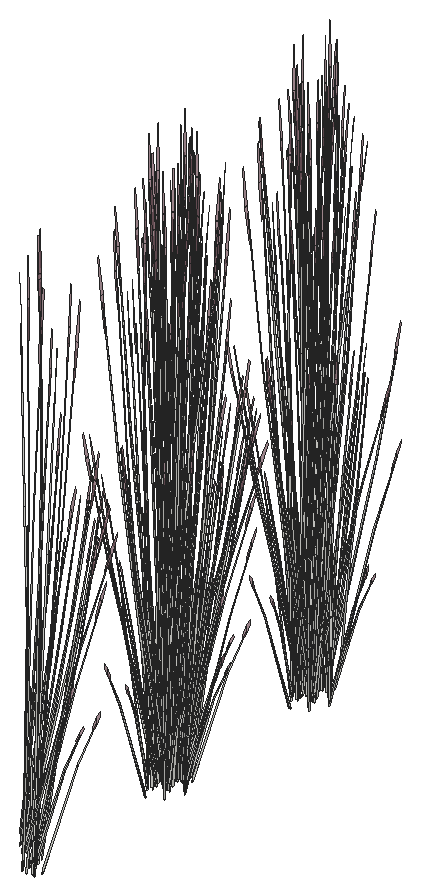
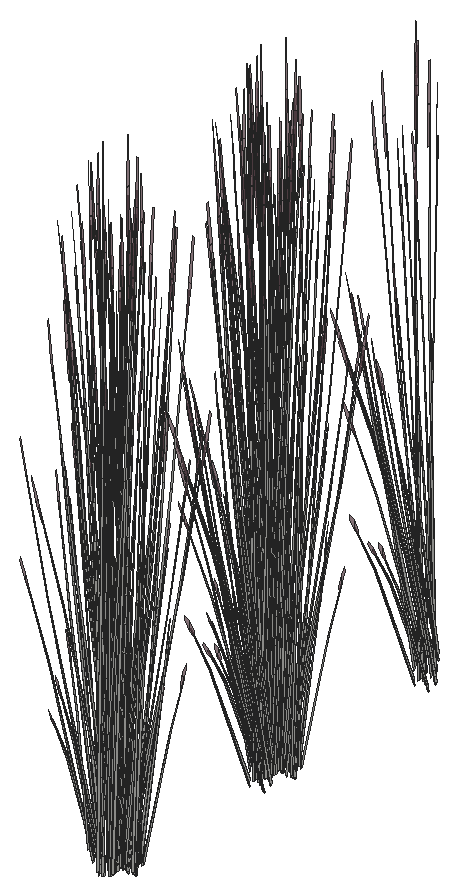
# SketchUp Ruby script. Lengths in inches.
U = 1.inch
M = Sketchup.active_model
def pt(a) = Geom::Point3d.new(a.map { |v| v * U })
def face(e, loops, mat)
  f = e.add_face(loops[0].map { |a| pt(a) })
  loops[1..].each { |l| e.add_face(l.map { |a| pt(a) }).erase! }
  f.material = f.back_material = mat if mat
  f
end
# faces: each face lists its corners as indices into pts; further lists are holes
def faces(e, pts, list, mat = nil) = list.each { |f| face(e, (f[0].is_a?(Array) ? f : [f]).map { |l| l.map { |i| pts[i] } }, mat) }
# xy, xz, yz: faces in a plane at the given z, y or x. An outline is a flat list of corners, or four numbers for a rectangle; further outlines are holes
def ring(l) = l.size == 4 ? [[l[0], l[1]], [l[2], l[1]], [l[2], l[3]], [l[0], l[3]]] : l.each_slice(2).to_a
def flat(e, list, mat, &to3) = list.each { |f| face(e, (f[0].is_a?(Array) ? f : [f]).map { |l| ring(l).map { |u, v| to3.(u, v) } }, mat) }
def xy(e, z, list, mat = nil) = flat(e, list, mat) { |x, y| [x, y, z] }
def xz(e, y, list, mat = nil) = flat(e, list, mat) { |x, z| [x, y, z] }
def yz(e, x, list, mat = nil) = flat(e, list, mat) { |y, z| [x, y, z] }
def lines(e, pts, list) = list.each { |a, b| e.add_line(pt(pts[a]), pt(pts[b])) }
# prism: a flat outline (further loops are holes) pulled along v
def prism(e, loops, v, mat = nil)
  f = face(e, loops, mat); d = Geom::Vector3d.new(v.map { |x| x * U })
  f.pushpull(f.normal.samedirection?(d) ? d.length : -d.length)
end
def box(e, o, s, mat = nil) = prism(e, [[o, [o[0] + s[0], o[1], o[2]], [o[0] + s[0], o[1] + s[1], o[2]], [o[0], o[1] + s[1], o[2]]]], [0, 0, s[2]], mat)
def at(x, y, z, deg = 0) = Geom::Transformation.translation(pt([x, y, z])) * Geom::Transformation.rotation(ORIGIN, Z_AXIS, deg.degrees)
def axes(o, x, y, z) = Geom::Transformation.new([*x, 0, *y, 0, *z, 0, *pt(o).to_a, 1])
def part(name) = M.definitions.add(name)
# library, detail: a bought-in or finely detailed component or shape, given as its bounding box
def library(name, o, s) = part(name).tap { |d| box(d.entities, o, s) }
def detail(e, o, s) = box(e.add_group.entities, o, s)
def put(e, d, t, mat = nil) = e.add_instance(d, t).tap { |i| i.material = mat if mat }
def group(e, t, mat = nil) = e.add_group.tap { |g| g.transformation = t; g.material = mat if mat }.entities
root = M.entities
M.materials.add("LightPink_Translucent").color = [144, 107, 117]
M.materials["LightPink_Translucent"].alpha = 0.75
c1 = part("blade")
p = [[2.15,0.21,22],[0,0.17,0],[0.09,0.45,0],[2.18,0.31,22],[2.29,0.31,22],[0.38,0.45,0],
  [2.48,0.24,33],[2.49,0.24,33],[2.48,0.22,33]]
faces(c1.entities,p,[[0,1,2,3],[4,5,2,3],[6,3,4,7],[8,0,3,6]])
c2 = part("seeds")
p = [[0.3,-0.1,1.38],[-0.01,-0.03,1.59],[-0.01,-0.03,0.03],[0.14,-0.07,-0.07],[0.29,-0.03,3],[0.15,0.01,3.11]]
faces(c2.entities,p,[[0,1,2,3],[1,0,4,5]],"LightPink_Translucent")
c3 = part("blade with seeds")
put(c3.entities,c1,at(0,0,0))
put(c3.entities,c2,axes([2.4,0.25,30.99],[1.5799,-0.05474,1.17369],[-0.12525,1.92788,0.29478],[-0.07173,-0.02425,1.56792]))
put(root,c3,axes([403.42,122.66,4.53],[0.20082,0.29199,-0.35414],[-0.2293,0.2764,0.4572],[0.1165,0.04206,0.87481]))
put(root,c3,axes([403.52,121.85,2.03],[-0.24637,0.29097,-0.30978],[-0.24637,-0.29097,0.30978],[0,0.09372,1.38974]))
put(root,c3,axes([402.46,121.88,2.67],[0.04113,0.53214,-0.29095],[-0.42835,0.03218,-0.50002],[-0.07543,0.07088,1.59708]))
put(root,c3,axes([402.61,121.67,2.21],[-0.17124,0.42022,-0.44739],[-0.35581,-0.20224,0.21531],[0,0.09687,1.43643]))
put(root,c3,axes([402.62,122.88,2.33],[0.44186,0.15158,0.30756],[-0.11054,0.54181,-0.36492],[-0.07313,0.06781,1.64885]))
put(root,c3,axes([402.59,123.24,2.02],[-0.33032,0.23318,-0.49651],[-0.19744,-0.41812,0],[-0.07523,0.05311,1.57504]))
put(root,c3,axes([403.6875,121.86,2.02],[0,0.46636,-0.49651],[-0.39487,0,0],[0,0.10622,1.57504]))
put(root,c3,axes([402.7,121.92,3.875],[-0.1311,-0.08035,1.71376],[0.27131,-0.33708,0.13857],[0.16909,0.15206,0.73262]))
put(root,c3,axes([403.18,122.83,2.77],[-0.19872,-0.13409,1.1486],[0.2566,-0.13625,0.84392],[0.06921,0.11541,0.25299]))
put(root,c3,axes([402.89,123.17,2.375],[0.22066,0.46731,0],[-0.36918,0.26061,-0.51607],[-0.08408,0.05936,1.63711]))
put(root,c3,axes([403.24,123.33,1.49],[0.02571,-0.06733,1.76342],[0.32373,-0.19829,-0.26939],[0.09815,0.10263,0.30037]))
put(root,c3,axes([402.7,121.32,2.84],[-0.00964,-0.43909,1.41272],[0.43635,0.11382,0.59816],[-0.1032,0.24027,1.3335]))
put(root,c3,axes([402.8125,121.8,2.09],[0.12941,0.42699,-0.69212],[-0.37279,0.15378,-0.18165],[0.0143,0.14459,1.52773]))
put(root,c3,axes([402.74,123.02,4.68],[0.34827,-0.11086,-0.51099],[0.06092,0.41983,-0.3958],[0.09354,0.12031,0.97773]))
put(root,c3,axes([403.22,123.44,2.67],[-0.22633,-0.01463,1.0506],[0.14947,-0.31064,0.58006],[0.08941,0.11036,0.8241]))
put(root,c3,axes([402.48,122.6875,2.59],[0.00623,-0.15459,1.43002],[0.29764,-0.17268,-0.30754],[0.09188,0.18503,0.61141]))
put(root,c3,axes([401.73,123.3125,1.49],[0.05712,-0.02538,1.76342],[0.34359,0.13968,-0.26939],[0.01005,0.15742,0.30037]))
put(root,c3,axes([401.21,122.91,5],[0.25266,0.31335,-0.5672],[-0.2669,0.27442,-0.43934],[-0.03844,0.15921,1.08528]))
put(root,c3,axes([400.9375,123.38,2.82],[0.32063,-0.08258,0.06507],[0.07371,0.33271,-0.86304],[-0.02033,0.16842,0.7736]))
put(root,c3,axes([401.96,123.21,4.68],[0.34695,0.11691,-0.51099],[-0.11892,0.40083,-0.3958],[0.03181,0.16138,0.97773]))
put(root,c3,axes([402.16,122.38,3.875],[-0.08068,-0.14973,1.71376],[0.3728,-0.12606,0.13857],[0.08426,0.23506,0.73262]))
put(root,c3,axes([401.8,123.46,4.53],[-0.1064,0.35863,-0.35414],[-0.31043,-0.1046,0.4572],[0.02846,0.14439,0.87481]))
put(root,c3,axes([401.5,122.46,3.875],[-0.00864,-0.17899,1.71376],[0.37441,0.11874,0.13857],[-0.02316,0.25508,0.73262]))
put(root,c3,axes([401.84,123.13,4.98],[0.16845,0.3792,-0.71045],[-0.34676,0.21133,0.08574],[0.03939,0.18322,1.00501]))
put(root,c3,axes([402.72,139.68,2.59],[-0.10032,0.0944,1.43002],[-0.30046,-0.16522,-0.30754],[0.05569,-0.20547,0.61141]))
put(root,c3,axes([402.27,140.01,4.98],[-0.16845,-0.3792,-0.71045],[0.34676,-0.21133,0.08574],[-0.03939,-0.18322,1.00501]))
put(root,c3,axes([401.98,139.17,1.49],[-0.0592,0.0168,1.76342],[-0.32738,-0.18913,-0.26939],[0.00549,-0.15776,0.30037]))
put(root,c3,axes([402.97,140.38,4.98],[0.00918,-0.43138,-0.71045],[0.38672,0.02897,0.08574],[0.04081,-0.18275,1.00501]))
put(root,c3,axes([402.3,139.6875,4.53],[0.1064,-0.35863,-0.35414],[0.31043,0.1046,0.4572],[-0.02846,-0.14439,0.87481]))
put(root,c3,axes([402.53,140.16,3.875],[-0.06572,0.16029,1.71376],[-0.27569,-0.33172,0.13857],[0.12437,-0.20675,0.73262]))
put(root,c3,axes([402.14,139.94,4.68],[-0.34695,-0.11691,-0.51099],[0.11892,-0.40083,-0.3958],[-0.03181,-0.16138,0.97773]))
put(root,c3,axes([402.35,138.93,2.77],[0.04528,0.27194,1.1486],[-0.25117,-0.15062,0.84392],[0.02703,-0.13924,0.25299]))
put(root,c3,axes([402.89,140.24,4.68],[-0.25266,-0.31335,-0.51099],[0.2669,-0.27442,-0.3958],[0.03844,-0.15921,0.97773]))
put(root,c3,axes([403.13,140.12,4.53],[0.23881,-0.24554,-0.35414],[0.22606,0.28036,0.4572],[0.0344,-0.14245,0.87481]))
put(root,c3,axes([401.49,141.4375,2.1],[-0.14494,-0.47823,-0.69835],[0.41752,-0.17223,-0.18329],[-0.01602,-0.16194,1.54149]))
put(root,c3,axes([403.43,139.97,1.49],[-0.05283,-0.03674,1.76342],[-0.13569,-0.41045,-0.26939],[0.09154,-0.11138,0.30037]))
put(root,c3,axes([403.42,141.13,4.98],[0.18436,-0.36797,-0.71045],[0.32306,0.26151,0.08574],[0.11008,-0.13332,1.00501]))
put(root,c3,axes([401.43,140.0625,2.375],[-0.22066,-0.46731,0],[0.36918,-0.26061,-0.51607],[0.08408,-0.05936,1.63711]))
put(root,c3,axes([403.41,140.96,4.68],[-0.09067,-0.42583,-0.51099],[0.34336,-0.07449,-0.3958],[0.0984,-0.11438,0.97773]))
put(root,c3,axes([401.92,139.5,2.13],[-0.2439,0.26754,-0.03893],[-0.22348,-0.29302,-0.17649],[-0.01573,-0.08303,0.58215]))
put(root,c3,axes([400.63,141.37,2.02],[0,-0.46636,-0.49651],[0.39487,0,0],[0,-0.10622,1.57504]))
put(root,c3,axes([401.73,139.99,2.02],[0.33032,-0.23318,-0.49651],[0.19744,0.41812,0],[0.07523,-0.05311,1.57504]))
put(root,c3,axes([403.69,140.79,2.59],[-0.12609,-0.01381,1.43002],[-0.12917,-0.37055,-0.30754],[0.1549,-0.10482,0.61141]))
put(root,c3,axes([402.12,140.94,2.06],[0.23773,-0.35053,-0.62353],[0.29532,0.31785,-0.16365],[0.09526,-0.08744,1.37633]))
put(root,c3,axes([403.84,140.11,2.77],[-0.11756,0.2374,1.1486],[-0.10105,-0.31895,0.84392],[0.09709,-0.07992,0.25299]))
put(root,c3,axes([403.67,141,4.53],[0.30722,-0.06665,-0.35414],[0.08112,0.381,0.4572],[0.08804,-0.10234,0.87481]))
put(root,c3,axes([401.71,141.56,2.21],[0.17124,-0.42022,-0.44739],[0.35581,0.20224,0.21531],[0,-0.09687,1.43643]))
put(root,c3,axes([401.86,141.35,2.67],[-0.04113,-0.53214,-0.29095],[0.42835,-0.03218,-0.50002],[0.07543,-0.07088,1.59708]))
put(root,c3,axes([400.8,141.38,2.03],[0.24637,-0.29097,-0.30978],[0.24637,0.29097,0.30978],[0,-0.09372,1.38974]))
put(root,c3,axes([401.67,141.91,2.67],[-0.39748,-0.22252,-0.29095],[0.19139,-0.46966,-0.50002],[-0.01249,-0.11531,1.59708]))
put(root,c3,axes([401.81,140.17,2.03],[0.32928,0.11539,-0.30978],[-0.08291,0.40636,0.30978],[0.06638,-0.04686,1.38974]))
put(root,c3,axes([401.92,141.77,2.43],[0.39767,0.22603,0.24065],[-0.19139,0.46966,0.50002],[0,-0.10827,1.60543]))
put(root,c3,axes([401.79,141.45,2.72],[-0.38326,0.02879,0.44739],[-0.03466,-0.47788,-0.21531],[0.06861,-0.04843,1.43643]))
put(root,c3,axes([400.8,141.8,2.48],[0,0.46636,0.49651],[-0.39487,0,0],[0,-0.10622,1.57504]))
put(root,c3,axes([403.57,141.91,4.68],[0.09562,-0.42421,-0.51099],[0.32782,0.1454,-0.3958],[0.13199,-0.0389,0.97773]))
put(root,c3,axes([403.06,140.18,2.375],[0.22066,-0.46731,0],[0.36918,0.26061,-0.51607],[0.08408,0.05936,1.63711]))
put(root,c3,axes([401.78,141.625,2.36],[0.15345,0.52148,0.45755],[-0.43845,0.18134,0.17955],[0.00536,-0.09582,1.58856]))
put(root,c3,axes([403.92,142.03,1.98],[-0.22732,0.05597,1.41583],[-0.03618,-0.44548,0.08104],[0.15921,-0.06743,0.80566]))
put(root,c3,axes([404.34,141.63,2.26],[-0.21881,-0.29821,-0.06488],[0.23965,-0.27324,-0.29416],[0.0679,-0.01924,0.97024]))
put(root,c3,axes([401.7,142.04,2.72],[-0.17124,0.42022,0.44739],[-0.35581,-0.20224,-0.21531],[0,-0.09687,1.43643]))
put(root,c3,axes([402.33,141.67,2.21],[0,-0.53961,0],[0.44133,0,0],[0,0,1.79456]))
put(root,c3,axes([402.87,140.42,2.48],[-0.33032,-0.23318,0.49651],[0.19744,-0.41812,0],[0.07523,0.05311,1.57504]))
put(root,c3,axes([403.51,142.06,4.98],[0.31014,-0.20596,-0.71045],[0.17284,0.42397,0.08574],[0.14985,-0.04816,1.00501]))
put(root,c3,axes([402.12,141.33,2.36],[-0.29264,0.42323,0.45755],[-0.34767,-0.3736,0.17955],[0.07055,-0.04224,1.58856]))
put(root,c3,axes([402.44,142.09,2.3],[-0.32829,-0.4014,-0.06131],[0.32849,-0.40164,0],[-0.01146,-0.01402,1.75571]))
put(root,c3,axes([401.61,140.63,2.47],[-0.10196,0.46348,0.17642],[-0.3731,-0.13116,0.35086],[0.06445,-0.00226,1.60407]))
put(root,c3,axes([401.46,141.01,1.59],[-0.3474,0.18671,1.28929],[-0.11057,-0.53572,0.50096],[0.21332,0.00891,1.46642]))
put(root,c3,axes([402.39,141.15,2.62],[0.06809,-0.4162,0.1448],[0.33266,0.07225,-0.41347],[0.06054,0.04274,1.26744]))
put(root,c3,axes([401.82,142.14,2.36],[0.44609,0.09826,0.45755],[-0.09078,0.55493,0.17955],[-0.06519,-0.05359,1.58856]))
put(root,c3,axes([404.17,141.73,1.49],[-0.01845,-0.0708,1.76342],[0.12793,-0.41416,-0.26939],[0.12905,-0.00596,0.30037]))
put(root,c3,axes([402.25,141.26,2.72],[-0.21202,-0.39143,0.44739],[0.32115,-0.27564,-0.21531],[0.06861,0.04843,1.43643]))
put(root,c3,axes([401.58,143.02,2.47],[0.37926,-0.12378,0.17642],[0.09365,0.46065,0.35086],[-0.03382,-0.06712,1.60407]))
put(root,c3,axes([402.36,141.28,2.67],[0.35635,-0.30962,-0.29095],[0.23697,0.43749,-0.50002],[0.08792,0.04443,1.59708]))
put(root,c3,axes([403.78,142.1,4.53],[0.29332,0.1301,-0.35414],[-0.08555,0.37955,0.4572],[0.11809,-0.0348,0.87481]))
put(root,c3,axes([403.26,140.46,2.02],[0.33032,0.23318,-0.49651],[-0.19744,0.41812,0],[0.07523,0.05311,1.57504]))
put(root,c3,axes([402.63,141.79,2.21],[0.39487,0,0],[0,0.48281,0],[0,0,1.78407]))
put(root,c3,axes([402.74,140.66,2.47],[-0.37926,0.12378,0.17642],[-0.09365,-0.46065,0.35086],[0.03382,0.06712,1.60407]))
put(root,c3,axes([402.98,141.63,3.875],[-0.14639,0.01056,1.71376],[0.09712,-0.45778,0.13857],[0.20862,0.02831,0.73262]))
put(root,c3,axes([403.17,140.63,2.03],[0.08291,0.40636,-0.30978],[-0.32928,0.11539,0.30978],[0.06638,0.04686,1.38974]))
put(root,c3,axes([402.5,141.54,2.38],[-0.44609,-0.09826,0.49198],[0.09078,-0.55493,0.19306],[0.06519,0.05359,1.70813]))
put(root,c3,axes([402.15,142.91,2.2],[-0.11516,-0.40207,0],[0.32884,-0.1408,0],[0,0,1.54371]))
put(root,c3,axes([401.93,142.53,2.62],[-0.06809,0.4162,0.1448],[-0.33266,-0.07225,-0.41347],[-0.06054,-0.04274,1.26744]))
put(root,c3,axes([402.58,142.86,2.18],[0.37054,-0.15823,-0.19198],[0.1302,0.45581,0.00008],[0.0409,-0.01749,1.73897]))
put(root,c3,axes([402.71,143.05,2.47],[0.10196,-0.46348,0.17642],[0.3731,0.13116,0.35086],[-0.06445,0.00226,1.60407]))
put(root,c3,axes([402.62,142,2.21],[0.24637,0.30123,0],[-0.24637,0.30123,0],[0,0,1.69266]))
put(root,c3,axes([403.29,141.87,2.47],[-0.2773,-0.3397,0.17642],[0.27945,-0.32949,0.35086],[-0.03063,0.06937,1.60407]))
put(root,c3,axes([402.78,141.35,2.06],[0.36714,0.07646,-0.62353],[-0.07747,0.47163,-0.16365],[0.10956,0.05715,1.37633]))
put(root,c3,axes([404.4,142.18,2.77],[-0.21807,0.07699,1.1486],[0.10265,-0.31819,0.84392],[0.11568,0.02177,0.25299]))
put(root,c3,axes([402.07,143.1,2.2],[-0.35581,-0.20937,0],[0.17124,-0.43505,0],[0,0,1.62707]))
put(root,c3,axes([402.62,141.64,2.72],[0.17124,-0.42022,0.44739],[0.35581,0.20224,-0.21531],[0,0.09687,1.43643]))
put(root,c3,axes([402.55,141.88,2.29],[0,0.53934,-0.05637],[-0.44133,0,0],[0,0.01695,1.79368]))
put(root,c3,axes([402.58,141.5,2.21],[0.21202,0.39143,-0.44739],[-0.32115,0.27564,0.21531],[0.06861,0.04843,1.43643]))
put(root,c3,axes([404.02,143.16,3.93],[-0.06755,-0.39203,-0.03492],[0.31928,-0.09013,-0.15832],[0.06667,0.02485,0.52218]))
put(root,c3,axes([403.52,141.88,2.48],[0,-0.46636,0.49651],[0.39487,0,0],[0,0.10622,1.57504]))
put(root,c3,axes([402.53,142.23,2.72],[0.38326,-0.02879,0.44739],[0.03466,0.47788,-0.21531],[-0.06861,0.04843,1.43643]))
put(root,c3,axes([402.77,141.74,2.62],[0.32884,-0.136,0.1448],[0.11516,0.38837,-0.41347],[0,0.08547,1.26744]))
put(root,c3,axes([403.99,142.6875,2.59],[-0.085,-0.1147,1.43002],[0.1106,-0.37943,-0.30754],[0.17198,0.0514,0.61141]))
put(root,c3,axes([402.47,143.1,2.2],[0.35581,0.20937,0],[-0.17124,0.43505,0],[0,0,1.74954]))
put(root,c3,axes([402.61,143.57,2.19],[-0.21791,-0.46895,-0.05142],[0.36918,-0.26061,0.51607],[-0.09097,0.04465,1.6363]))
put(root,c3,axes([402.53,142.43,2.62],[0.26075,0.2802,0.1448],[-0.2175,0.31612,-0.41347],[-0.06054,0.04274,1.26744]))
put(root,c3,axes([403.21,142.92,4.98],[0.35281,0.01123,-0.71045],[-0.0237,0.47284,0.08574],[0.14947,0.0499,1.00501]))
put(root,c3,axes([402.8125,143.3,2.48],[0.33032,-0.23318,0.49651],[0.19744,0.41812,0],[-0.07523,0.05311,1.57504]))
put(root,c3,axes([402.34,142.93,2.29],[0.15345,0.53576,-0.06012],[-0.43845,0.18773,0],[0.00536,0.01871,1.72173]))
put(root,c3,axes([402.51,143.51,2.03],[-0.32928,-0.11539,-0.30978],[0.08291,-0.40636,0.30978],[-0.06638,0.04686,1.38974]))
put(root,c3,axes([403.78,141.96,2.375],[0.44133,0,0],[0,0.52122,-0.51607],[0,0.11871,1.63711]))
put(root,c3,axes([403.61,142.23,2.2],[-0.44111,-0.00373,-0.04976],[0,-0.52122,0.49943],[-0.01386,0.11865,1.58352]))
put(root,c3,axes([402.65,141.77,2.67],[0.39748,0.22252,-0.29095],[-0.19139,0.46966,-0.50002],[0.01249,0.11531,1.59708]))
put(root,c3,axes([403.42,143.11,4.53],[0.20082,0.29199,-0.35414],[-0.2293,0.2764,0.4572],[0.1165,0.04206,0.87481]))
put(root,c3,axes([403.52,142.3,2.03],[-0.24637,0.29097,-0.30978],[-0.24637,-0.29097,0.30978],[0,0.09372,1.38974]))
put(root,c3,axes([402.46,142.33,2.67],[0.04113,0.53214,-0.29095],[-0.42835,0.03218,-0.50002],[-0.07543,0.07088,1.59708]))
put(root,c3,axes([402.61,142.12,2.21],[-0.17124,0.42022,-0.44739],[-0.35581,-0.20224,0.21531],[0,0.09687,1.43643]))
put(root,c3,axes([402.62,143.33,2.33],[0.44186,0.15158,0.30756],[-0.11054,0.54181,-0.36492],[-0.07313,0.06781,1.64885]))
put(root,c3,axes([402.59,143.69,2.02],[-0.33032,0.23318,-0.49651],[-0.19744,-0.41812,0],[-0.07523,0.05311,1.57504]))
put(root,c3,axes([403.6875,142.3125,2.02],[0,0.46636,-0.49651],[-0.39487,0,0],[0,0.10622,1.57504]))
put(root,c3,axes([402.7,142.36,3.875],[-0.1311,-0.08035,1.71376],[0.27131,-0.33708,0.13857],[0.16909,0.15206,0.73262]))
put(root,c3,axes([403.18,143.28,2.77],[-0.19872,-0.13409,1.1486],[0.2566,-0.13625,0.84392],[0.06921,0.11541,0.25299]))
put(root,c3,axes([402.89,143.62,2.375],[0.22066,0.46731,0],[-0.36918,0.26061,-0.51607],[-0.08408,0.05936,1.63711]))
put(root,c3,axes([403.24,143.78,1.49],[0.02571,-0.06733,1.76342],[0.32373,-0.19829,-0.26939],[0.09815,0.10263,0.30037]))
put(root,c3,axes([402.7,141.77,2.84],[-0.00964,-0.43909,1.41272],[0.43635,0.11382,0.59816],[-0.1032,0.24027,1.3335]))
put(root,c3,axes([402.8125,142.25,2.09],[0.12941,0.42699,-0.69212],[-0.37279,0.15378,-0.18165],[0.0143,0.14459,1.52773]))
put(root,c3,axes([402.74,143.46,4.68],[0.34827,-0.11086,-0.51099],[0.06092,0.41983,-0.3958],[0.09354,0.12031,0.97773]))
put(root,c3,axes([403.22,143.89,2.67],[-0.22633,-0.01463,1.0506],[0.14947,-0.31064,0.58006],[0.08941,0.11036,0.8241]))
put(root,c3,axes([402.48,143.14,2.59],[0.00623,-0.15459,1.43002],[0.29764,-0.17268,-0.30754],[0.09188,0.18503,0.61141]))
put(root,c3,axes([401.73,143.76,1.49],[0.05712,-0.02538,1.76342],[0.34359,0.13968,-0.26939],[0.01005,0.15742,0.30037]))
put(root,c3,axes([401.21,143.36,5],[0.25266,0.31335,-0.5672],[-0.2669,0.27442,-0.43934],[-0.03844,0.15921,1.08528]))
put(root,c3,axes([400.9375,143.83,2.82],[0.32063,-0.08258,0.06507],[0.07371,0.33271,-0.86304],[-0.02033,0.16842,0.7736]))
put(root,c3,axes([401.96,143.66,4.68],[0.34695,0.11691,-0.51099],[-0.11892,0.40083,-0.3958],[0.03181,0.16138,0.97773]))
put(root,c3,axes([402.16,142.83,3.875],[-0.08068,-0.14973,1.71376],[0.3728,-0.12606,0.13857],[0.08426,0.23506,0.73262]))
put(root,c3,axes([401.8,143.9,4.53],[-0.1064,0.35863,-0.35414],[-0.31043,-0.1046,0.4572],[0.02846,0.14439,0.87481]))
put(root,c3,axes([401.5,142.91,3.875],[-0.00864,-0.17899,1.71376],[0.37441,0.11874,0.13857],[-0.02316,0.25508,0.73262]))
put(root,c3,axes([401.84,143.58,4.98],[0.16845,0.3792,-0.71045],[-0.34676,0.21133,0.08574],[0.03939,0.18322,1.00501]))
put(root,c3,axes([402.72,159.38,2.59],[-0.10032,0.0944,1.43002],[-0.30046,-0.16522,-0.30754],[0.05569,-0.20547,0.61141]))
put(root,c3,axes([402.27,159.71,4.98],[-0.16845,-0.3792,-0.71045],[0.34676,-0.21133,0.08574],[-0.03939,-0.18322,1.00501]))
put(root,c3,axes([401.98,158.86,1.49],[-0.0592,0.0168,1.76342],[-0.32738,-0.18913,-0.26939],[0.00549,-0.15776,0.30037]))
put(root,c3,axes([402.97,160.08,4.98],[0.00918,-0.43138,-0.71045],[0.38672,0.02897,0.08574],[0.04081,-0.18275,1.00501]))
put(root,c3,axes([402.3,159.38,4.53],[0.1064,-0.35863,-0.35414],[0.31043,0.1046,0.4572],[-0.02846,-0.14439,0.87481]))
put(root,c3,axes([402.53,159.86,3.875],[-0.06572,0.16029,1.71376],[-0.27569,-0.33172,0.13857],[0.12437,-0.20675,0.73262]))
put(root,c3,axes([402.14,159.63,4.68],[-0.34695,-0.11691,-0.51099],[0.11892,-0.40083,-0.3958],[-0.03181,-0.16138,0.97773]))
put(root,c3,axes([402.35,158.625,2.77],[0.04528,0.27194,1.1486],[-0.25117,-0.15062,0.84392],[0.02703,-0.13924,0.25299]))
put(root,c3,axes([402.89,159.93,4.68],[-0.25266,-0.31335,-0.51099],[0.2669,-0.27442,-0.3958],[0.03844,-0.15921,0.97773]))
put(root,c3,axes([403.13,159.82,4.53],[0.23881,-0.24554,-0.35414],[0.22606,0.28036,0.4572],[0.0344,-0.14245,0.87481]))
put(root,c3,axes([401.49,161.13,2.1],[-0.14494,-0.47823,-0.69835],[0.41752,-0.17223,-0.18329],[-0.01602,-0.16194,1.54149]))
put(root,c3,axes([403.43,159.67,1.49],[-0.05283,-0.03674,1.76342],[-0.13569,-0.41045,-0.26939],[0.09154,-0.11138,0.30037]))
put(root,c3,axes([403.42,160.83,4.98],[0.18436,-0.36797,-0.71045],[0.32306,0.26151,0.08574],[0.11008,-0.13332,1.00501]))
put(root,c3,axes([401.43,159.75,2.375],[-0.22066,-0.46731,0],[0.36918,-0.26061,-0.51607],[0.08408,-0.05936,1.63711]))
put(root,c3,axes([403.41,160.65,4.68],[-0.09067,-0.42583,-0.51099],[0.34336,-0.07449,-0.3958],[0.0984,-0.11438,0.97773]))
put(root,c3,axes([401.92,159.19,2.13],[-0.2439,0.26754,-0.03893],[-0.22348,-0.29302,-0.17649],[-0.01573,-0.08303,0.58215]))
put(root,c3,axes([400.63,161.0625,2.02],[0,-0.46636,-0.49651],[0.39487,0,0],[0,-0.10622,1.57504]))
put(root,c3,axes([401.73,159.68,2.02],[0.33032,-0.23318,-0.49651],[0.19744,0.41812,0],[0.07523,-0.05311,1.57504]))
put(root,c3,axes([403.69,160.49,2.59],[-0.12609,-0.01381,1.43002],[-0.12917,-0.37055,-0.30754],[0.1549,-0.10482,0.61141]))
put(root,c3,axes([402.12,160.64,2.06],[0.23773,-0.35053,-0.62353],[0.29532,0.31785,-0.16365],[0.09526,-0.08744,1.37633]))
put(root,c3,axes([403.84,159.81,2.77],[-0.11756,0.2374,1.1486],[-0.10105,-0.31895,0.84392],[0.09709,-0.07992,0.25299]))
put(root,c3,axes([403.67,160.7,4.53],[0.30722,-0.06665,-0.35414],[0.08112,0.381,0.4572],[0.08804,-0.10234,0.87481]))
put(root,c3,axes([401.71,161.25,2.21],[0.17124,-0.42022,-0.44739],[0.35581,0.20224,0.21531],[0,-0.09687,1.43643]))
put(root,c3,axes([401.86,161.05,2.67],[-0.04113,-0.53214,-0.29095],[0.42835,-0.03218,-0.50002],[0.07543,-0.07088,1.59708]))
put(root,c3,axes([400.8,161.07,2.03],[0.24637,-0.29097,-0.30978],[0.24637,0.29097,0.30978],[0,-0.09372,1.38974]))
put(root,c3,axes([401.67,161.6,2.67],[-0.39748,-0.22252,-0.29095],[0.19139,-0.46966,-0.50002],[-0.01249,-0.11531,1.59708]))
put(root,c3,axes([401.81,159.87,2.03],[0.32928,0.11539,-0.30978],[-0.08291,0.40636,0.30978],[0.06638,-0.04686,1.38974]))
put(root,c3,axes([401.92,161.46,2.43],[0.39767,0.22603,0.24065],[-0.19139,0.46966,0.50002],[0,-0.10827,1.60543]))
put(root,c3,axes([401.77,162.1,2.4375],[0.09355,-0.55261,-0.23429],[0.44354,0.09633,0.51271],[-0.0775,-0.07631,1.5644]))
put(root,c3,axes([401.79,161.15,2.72],[-0.38326,0.02879,0.44739],[-0.03466,-0.47788,-0.21531],[0.06861,-0.04843,1.43643]))
put(root,c3,axes([400.8,161.5,2.48],[0,0.46636,0.49651],[-0.39487,0,0],[0,-0.10622,1.57504]))
put(root,c3,axes([403.57,161.6,4.68],[0.09562,-0.42421,-0.51099],[0.32782,0.1454,-0.3958],[0.13199,-0.0389,0.97773]))
put(root,c3,axes([403.06,159.87,2.375],[0.22066,-0.46731,0],[0.36918,0.26061,-0.51607],[0.08408,0.05936,1.63711]))
put(root,c3,axes([401.78,161.32,2.36],[0.15345,0.52148,0.45755],[-0.43845,0.18134,0.17955],[0.00536,-0.09582,1.58856]))
put(root,c3,axes([403.92,161.72,1.98],[-0.22732,0.05597,1.41583],[-0.03618,-0.44548,0.08104],[0.15921,-0.06743,0.80566]))
put(root,c3,axes([404.34,161.32,2.26],[-0.21881,-0.29821,-0.06488],[0.23965,-0.27324,-0.29416],[0.0679,-0.01924,0.97024]))
put(root,c3,axes([401.7,161.73,2.72],[-0.17124,0.42022,0.44739],[-0.35581,-0.20224,-0.21531],[0,-0.09687,1.43643]))
put(root,c3,axes([402.33,161.36,2.21],[0,-0.53961,0],[0.44133,0,0],[0,0,1.79456]))
put(root,c3,axes([402.87,160.12,2.48],[-0.33032,-0.23318,0.49651],[0.19744,-0.41812,0],[0.07523,0.05311,1.57504]))
put(root,c3,axes([403.51,161.75,4.98],[0.31014,-0.20596,-0.71045],[0.17284,0.42397,0.08574],[0.14985,-0.04816,1.00501]))
put(root,c3,axes([402.12,161.02,2.36],[-0.29264,0.42323,0.45755],[-0.34767,-0.3736,0.17955],[0.07055,-0.04224,1.58856]))
put(root,c3,axes([402.44,161.78,2.3],[-0.32829,-0.4014,-0.06131],[0.32849,-0.40164,0],[-0.01146,-0.01402,1.75571]))
put(root,c3,axes([401.61,160.33,2.47],[-0.10196,0.46348,0.17642],[-0.3731,-0.13116,0.35086],[0.06445,-0.00226,1.60407]))
put(root,c3,axes([401.46,160.7,1.59],[-0.3474,0.18671,1.28929],[-0.11057,-0.53572,0.50096],[0.21332,0.00891,1.46642]))
put(root,c3,axes([402.39,160.84,2.62],[0.06809,-0.4162,0.1448],[0.33266,0.07225,-0.41347],[0.06054,0.04274,1.26744]))
put(root,c3,axes([401.82,161.83,2.36],[0.44609,0.09826,0.45755],[-0.09078,0.55493,0.17955],[-0.06519,-0.05359,1.58856]))
put(root,c3,axes([404.17,161.43,1.49],[-0.01845,-0.0708,1.76342],[0.12793,-0.41416,-0.26939],[0.12905,-0.00596,0.30037]))
put(root,c3,axes([402.25,160.95,2.72],[-0.21202,-0.39143,0.44739],[0.32115,-0.27564,-0.21531],[0.06861,0.04843,1.43643]))
put(root,c3,axes([401.58,162.72,2.47],[0.37926,-0.12378,0.17642],[0.09365,0.46065,0.35086],[-0.03382,-0.06712,1.60407]))
put(root,c3,axes([402.36,160.98,2.67],[0.35635,-0.30962,-0.29095],[0.23697,0.43749,-0.50002],[0.08792,0.04443,1.59708]))
put(root,c3,axes([403.78,161.79,4.53],[0.29332,0.1301,-0.35414],[-0.08555,0.37955,0.4572],[0.11809,-0.0348,0.87481]))
put(root,c3,axes([403.26,160.15,2.02],[0.33032,0.23318,-0.49651],[-0.19744,0.41812,0],[0.07523,0.05311,1.57504]))
put(root,c3,axes([402.63,161.48,2.21],[0.39487,0,0],[0,0.48281,0],[0,0,1.78407]))
put(root,c3,axes([402.74,160.35,2.47],[-0.37926,0.12378,0.17642],[-0.09365,-0.46065,0.35086],[0.03382,0.06712,1.60407]))
put(root,c3,axes([402.98,161.32,3.875],[-0.14639,0.01056,1.71376],[0.09712,-0.45778,0.13857],[0.20862,0.02831,0.73262]))
put(root,c3,axes([403.17,160.33,2.03],[0.08291,0.40636,-0.30978],[-0.32928,0.11539,0.30978],[0.06638,0.04686,1.38974]))
put(root,c3,axes([402.5,161.24,2.38],[-0.44609,-0.09826,0.49198],[0.09078,-0.55493,0.19306],[0.06519,0.05359,1.70813]))
put(root,c3,axes([402.15,162.61,2.2],[-0.11516,-0.40207,0],[0.32884,-0.1408,0],[0,0,1.54371]))
put(root,c3,axes([401.93,162.23,2.62],[-0.06809,0.4162,0.1448],[-0.33266,-0.07225,-0.41347],[-0.06054,-0.04274,1.26744]))
put(root,c3,axes([402.58,162.55,2.18],[0.37054,-0.15823,-0.19198],[0.1302,0.45581,0.00008],[0.0409,-0.01749,1.73897]))
put(root,c3,axes([402.71,162.74,2.47],[0.10196,-0.46348,0.17642],[0.3731,0.13116,0.35086],[-0.06445,0.00226,1.60407]))
put(root,c3,axes([402.62,161.69,2.21],[0.24637,0.30123,0],[-0.24637,0.30123,0],[0,0,1.69266]))
put(root,c3,axes([403.29,161.56,2.47],[-0.2773,-0.3397,0.17642],[0.27945,-0.32949,0.35086],[-0.03063,0.06937,1.60407]))
put(root,c3,axes([402.78,161.05,2.06],[0.36714,0.07646,-0.62353],[-0.07747,0.47163,-0.16365],[0.10956,0.05715,1.37633]))
put(root,c3,axes([404.4,161.87,2.77],[-0.21807,0.07699,1.1486],[0.10265,-0.31819,0.84392],[0.11568,0.02177,0.25299]))
put(root,c3,axes([402.07,162.79,2.2],[-0.35581,-0.20937,0],[0.17124,-0.43505,0],[0,0,1.62707]))
put(root,c3,axes([402.62,161.34,2.72],[0.17124,-0.42022,0.44739],[0.35581,0.20224,-0.21531],[0,0.09687,1.43643]))
put(root,c3,axes([402.55,161.58,2.29],[0,0.53934,-0.05637],[-0.44133,0,0],[0,0.01695,1.79368]))
put(root,c3,axes([402.58,161.2,2.21],[0.21202,0.39143,-0.44739],[-0.32115,0.27564,0.21531],[0.06861,0.04843,1.43643]))
put(root,c3,axes([404.02,162.85,3.93],[-0.06755,-0.39203,-0.03492],[0.31928,-0.09013,-0.15832],[0.06667,0.02485,0.52218]))
put(root,c3,axes([403.52,161.57,2.48],[0,-0.46636,0.49651],[0.39487,0,0],[0,0.10622,1.57504]))
put(root,c3,axes([402.53,161.92,2.72],[0.38326,-0.02879,0.44739],[0.03466,0.47788,-0.21531],[-0.06861,0.04843,1.43643]))
put(root,c3,axes([402.77,161.43,2.62],[0.32884,-0.136,0.1448],[0.11516,0.38837,-0.41347],[0,0.08547,1.26744]))
put(root,c3,axes([403.99,162.38,2.59],[-0.085,-0.1147,1.43002],[0.1106,-0.37943,-0.30754],[0.17198,0.0514,0.61141]))
put(root,c3,axes([402.47,162.8,2.2],[0.35581,0.20937,0],[-0.17124,0.43505,0],[0,0,1.74954]))
put(root,c3,axes([402.61,163.26,2.19],[-0.21791,-0.46895,-0.05142],[0.36918,-0.26061,0.51607],[-0.09097,0.04465,1.6363]))
put(root,c3,axes([402.53,162.13,2.62],[0.26075,0.2802,0.1448],[-0.2175,0.31612,-0.41347],[-0.06054,0.04274,1.26744]))
put(root,c3,axes([403.21,162.61,4.98],[0.35281,0.01123,-0.71045],[-0.0237,0.47284,0.08574],[0.14947,0.0499,1.00501]))
put(root,c3,axes([402.8125,162.99,2.48],[0.33032,-0.23318,0.49651],[0.19744,0.41812,0],[-0.07523,0.05311,1.57504]))
